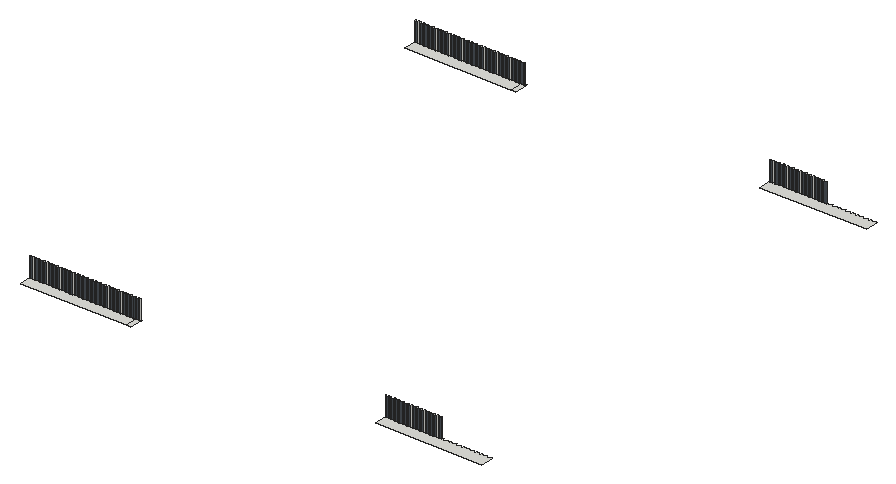
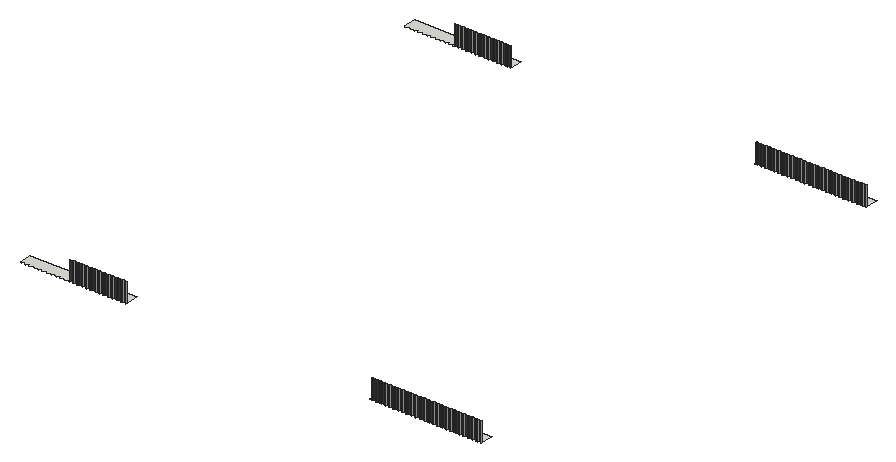
# SketchUp Ruby script. Lengths in inches.
U = 1.inch
M = Sketchup.active_model
def pt(a) = Geom::Point3d.new(a.map { |v| v * U })
def face(e, loops, mat)
  f = e.add_face(loops[0].map { |a| pt(a) })
  loops[1..].each { |l| e.add_face(l.map { |a| pt(a) }).erase! }
  f.material = f.back_material = mat if mat
  f
end
# faces: each face lists its corners as indices into pts; further lists are holes
def faces(e, pts, list, mat = nil) = list.each { |f| face(e, (f[0].is_a?(Array) ? f : [f]).map { |l| l.map { |i| pts[i] } }, mat) }
# xy, xz, yz: faces in a plane at the given z, y or x. An outline is a flat list of corners, or four numbers for a rectangle; further outlines are holes
def ring(l) = l.size == 4 ? [[l[0], l[1]], [l[2], l[1]], [l[2], l[3]], [l[0], l[3]]] : l.each_slice(2).to_a
def flat(e, list, mat, &to3) = list.each { |f| face(e, (f[0].is_a?(Array) ? f : [f]).map { |l| ring(l).map { |u, v| to3.(u, v) } }, mat) }
def xy(e, z, list, mat = nil) = flat(e, list, mat) { |x, y| [x, y, z] }
def xz(e, y, list, mat = nil) = flat(e, list, mat) { |x, z| [x, y, z] }
def yz(e, x, list, mat = nil) = flat(e, list, mat) { |y, z| [x, y, z] }
def lines(e, pts, list) = list.each { |a, b| e.add_line(pt(pts[a]), pt(pts[b])) }
# prism: a flat outline (further loops are holes) pulled along v
def prism(e, loops, v, mat = nil)
  f = face(e, loops, mat); d = Geom::Vector3d.new(v.map { |x| x * U })
  f.pushpull(f.normal.samedirection?(d) ? d.length : -d.length)
end
def box(e, o, s, mat = nil) = prism(e, [[o, [o[0] + s[0], o[1], o[2]], [o[0] + s[0], o[1] + s[1], o[2]], [o[0], o[1] + s[1], o[2]]]], [0, 0, s[2]], mat)
def at(x, y, z, deg = 0) = Geom::Transformation.translation(pt([x, y, z])) * Geom::Transformation.rotation(ORIGIN, Z_AXIS, deg.degrees)
def axes(o, x, y, z) = Geom::Transformation.new([*x, 0, *y, 0, *z, 0, *pt(o).to_a, 1])
def part(name) = M.definitions.add(name)
# library, detail: a bought-in or finely detailed component or shape, given as its bounding box
def library(name, o, s) = part(name).tap { |d| box(d.entities, o, s) }
def detail(e, o, s) = box(e.add_group.entities, o, s)
def put(e, d, t, mat = nil) = e.add_instance(d, t).tap { |i| i.material = mat if mat }
def group(e, t, mat = nil) = e.add_group.tap { |g| g.transformation = t; g.material = mat if mat }.entities
root = M.entities
M.materials.add("[Formica Blue]").color = [73, 80, 86]
xy(root,693.65,[[137.5,412.04,353.97,412.04,353.97,437.1,352.41,437.1,352.41,438.72,349.85,438.72,349.85,437.1,343.52,437.1,343.52,438.72,340.96,438.72,340.96,437.1,334.63,437.1,334.63,438.72,332.07,438.72,332.07,437.1,325.74,437.1,325.74,438.72,323.18,438.72,323.18,437.1,316.85,437.1,316.85,438.72,314.29,438.72,314.29,437.1,307.95,437.1,307.95,438.72,305.4,438.72,305.4,437.1,299.0625,437.1,299.0625,438.72,296.51,438.72,296.51,437.1,290.17,437.1,290.17,438.72,287.61,438.72,287.61,437.1,281.28,437.1,281.28,438.72,278.72,438.72,278.72,437.1,272.39,437.1,272.39,438.72,269.83,438.72,269.83,437.1,263.5,437.1,263.5,438.72,260.94,438.72,260.94,437.1,254.61,437.1,254.61,438.72,252.05,438.72,252.05,437.1,245.72,437.1,245.72,438.72,243.16,438.72,243.16,437.1,236.82,437.1,236.82,438.72,234.27,438.72,234.27,437.1,227.93,437.1,227.93,438.72,225.375,438.72,225.375,437.1,219.04,437.1,219.04,438.72,216.48,438.72,216.48,437.1,210.15,437.1,210.15,438.72,207.59,438.72,207.59,437.1,201.26,437.1,201.26,438.72,198.7,438.72,198.7,437.1,192.37,437.1,192.37,438.72,189.81,438.72,189.81,437.1,183.48,437.1,183.48,438.72,180.92,438.72,180.92,437.1,174.59,437.1,174.59,438.72,172.03,438.72,172.03,437.1,165.69,437.1,165.69,438.72,163.14,438.72,163.14,437.1,156.8,437.1,156.8,438.72,154.24,438.72,154.24,437.1,147.91,437.1,147.91,438.72,143.93,438.72,143.93,437.1,137.6,437.1,137.6,438.72,137.5,438.72],[353.97,412.04,363.73,412.04,363.73,437.1,361.3,437.1,361.3,438.72,358.74,438.72,358.74,437.1,353.97,437.1],[861.9375,412.04,1078.41,412.04,1078.41,437.1,1076.85,437.1,1076.85,438.72,1074.29,438.72,1074.29,437.1,1067.96,437.1,1067.96,438.72,1065.4,438.72,1065.4,437.1,1059.07,437.1,1059.07,438.72,1056.51,438.72,1056.51,437.1,1050.17,437.1,1050.17,438.72,1047.62,438.72,1047.62,437.1,1041.28,437.1,1041.28,438.72,1038.73,438.72,1038.73,437.1,1032.39,437.1,1032.39,438.72,1029.83,438.72,1029.83,437.1,1023.5,437.1,1023.5,438.72,1020.94,438.72,1020.94,437.1,1014.61,437.1,1014.61,438.72,1012.05,438.72,1012.05,437.1,1005.72,437.1,1005.72,438.72,1003.16,438.72,1003.16,437.1,996.83,437.1,996.83,438.72,994.27,438.72,994.27,437.1,987.9375,437.1,987.9375,438.72,985.38,438.72,985.38,437.1,979.04,437.1,979.04,438.72,976.49,438.72,976.49,437.1,970.15,437.1,970.15,438.72,967.6,438.72,967.6,437.1,961.26,437.1,961.26,438.72,958.7,438.72,958.7,437.1,952.37,437.1,952.37,438.72,949.8125,438.72,949.8125,437.1,943.48,437.1,943.48,438.72,940.92,438.72,940.92,437.1,934.59,437.1,934.59,438.72,932.03,438.72,932.03,437.1,925.7,437.1,925.7,438.72,923.14,438.72,923.14,437.1,916.81,437.1,916.81,438.72,914.25,438.72,914.25,437.1,907.91,437.1,907.91,438.72,905.36,438.72,905.36,437.1,899.02,437.1,899.02,438.72,896.47,438.72,896.47,437.1,890.13,437.1,890.13,438.72,887.57,438.72,887.57,437.1,881.24,437.1,881.24,438.72,878.68,438.72,878.68,437.1,872.35,437.1,872.35,438.72,868.37,438.72,868.37,437.1,862.04,437.1,862.04,438.72,861.9375,438.72],[361.3,437.1,363.73,438.72],[137.5,1392.39,353.97,1392.39,353.97,1417.45,352.41,1417.45,352.41,1419.07,349.85,1419.07,349.85,1417.45,343.52,1417.45,343.52,1419.07,340.96,1419.07,340.96,1417.45,334.63,1417.45,334.63,1419.07,332.07,1419.07,332.07,1417.45,325.74,1417.45,325.74,1419.07,323.18,1419.07,323.18,1417.45,316.85,1417.45,316.85,1419.07,314.29,1419.07,314.29,1417.45,307.95,1417.45,307.95,1419.07,305.4,1419.07,305.4,1417.45,299.0625,1417.45,299.0625,1419.07,296.51,1419.07,296.51,1417.45,290.17,1417.45,290.17,1419.07,287.61,1419.07,287.61,1417.45,281.28,1417.45,281.28,1419.07,278.72,1419.07,278.72,1417.45,272.39,1417.45,272.39,1419.07,269.83,1419.07,269.83,1417.45,263.5,1417.45,263.5,1419.07,260.94,1419.07,260.94,1417.45,254.61,1417.45,254.61,1419.07,252.05,1419.07,252.05,1417.45,245.72,1417.45,245.72,1419.07,243.16,1419.07,243.16,1417.45,236.82,1417.45,236.82,1419.07,234.27,1419.07,234.27,1417.45,227.93,1417.45,227.93,1419.07,225.375,1419.07,225.375,1417.45,219.04,1417.45,219.04,1419.07,216.48,1419.07,216.48,1417.45,210.15,1417.45,210.15,1419.07,207.59,1419.07,207.59,1417.45,201.26,1417.45,201.26,1419.07,198.7,1419.07,198.7,1417.45,192.37,1417.45,192.37,1419.07,189.81,1419.07,189.81,1417.45,183.48,1417.45,183.48,1419.07,180.92,1419.07,180.92,1417.45,174.59,1417.45,174.59,1419.07,172.03,1419.07,172.03,1417.45,165.69,1417.45,165.69,1419.07,163.14,1419.07,163.14,1417.45,156.8,1417.45,156.8,1419.07,154.24,1419.07,154.24,1417.45,147.91,1417.45,147.91,1419.07,143.93,1419.07,143.93,1417.45,137.6,1417.45,137.6,1419.07,137.5,1419.07],
  [353.97,1392.39,363.73,1392.39,363.73,1417.45,361.3,1417.45,361.3,1419.07,358.74,1419.07,358.74,1417.45,353.97,1417.45],[861.9375,1392.39,1078.41,1392.39,1078.41,1417.45,1076.85,1417.45,1076.85,1419.07,1074.29,1419.07,1074.29,1417.45,1067.96,1417.45,1067.96,1419.07,1065.4,1419.07,1065.4,1417.45,1059.07,1417.45,1059.07,1419.07,1056.51,1419.07,1056.51,1417.45,1050.17,1417.45,1050.17,1419.07,1047.62,1419.07,1047.62,1417.45,1041.28,1417.45,1041.28,1419.07,1038.73,1419.07,1038.73,1417.45,1032.39,1417.45,1032.39,1419.07,1029.83,1419.07,1029.83,1417.45,1023.5,1417.45,1023.5,1419.07,1020.94,1419.07,1020.94,1417.45,1014.61,1417.45,1014.61,1419.07,1012.05,1419.07,1012.05,1417.45,1005.72,1417.45,1005.72,1419.07,1003.16,1419.07,1003.16,1417.45,996.83,1417.45,996.83,1419.07,994.27,1419.07,994.27,1417.45,987.9375,1417.45,987.9375,1419.07,985.38,1419.07,985.38,1417.45,979.04,1417.45,979.04,1419.07,976.49,1419.07,976.49,1417.45,970.15,1417.45,970.15,1419.07,967.6,1419.07,967.6,1417.45,961.26,1417.45,961.26,1419.07,958.7,1419.07,958.7,1417.45,952.37,1417.45,952.37,1419.07,949.8125,1419.07,949.8125,1417.45,943.48,1417.45,943.48,1419.07,940.92,1419.07,940.92,1417.45,934.59,1417.45,934.59,1419.07,932.03,1419.07,932.03,1417.45,925.7,1417.45,925.7,1419.07,923.14,1419.07,923.14,1417.45,916.81,1417.45,916.81,1419.07,914.25,1419.07,914.25,1417.45,907.91,1417.45,907.91,1419.07,905.36,1419.07,905.36,1417.45,899.02,1417.45,899.02,1419.07,896.47,1419.07,896.47,1417.45,890.13,1417.45,890.13,1419.07,887.57,1419.07,887.57,1417.45,881.24,1417.45,881.24,1419.07,878.68,1419.07,878.68,1417.45,872.35,1417.45,872.35,1419.07,868.37,1419.07,868.37,1417.45,862.04,1417.45,862.04,1419.07,861.9375,1419.07],[361.3,1417.45,363.73,1419.07]])
xz(root,437.1,[[137.6,693.65,143.93,733.125],[147.91,693.65,154.24,733.125],[156.8,693.65,163.14,733.125],[165.69,693.65,172.03,733.125],[174.59,693.65,180.92,733.125],
  [183.48,693.65,189.81,733.125],[192.37,693.65,198.7,733.125],[201.26,693.65,207.59,733.125],[210.15,693.65,216.48,733.125],[219.04,693.65,225.375,733.125],
  [227.93,693.65,234.27,733.125],[236.82,693.65,243.16,733.125],[245.72,693.65,252.05,733.125],[254.61,693.65,260.94,733.125],[263.5,693.65,269.83,733.125],
  [272.39,693.65,278.72,733.125],[281.28,693.65,287.61,733.125],[290.17,693.65,296.51,733.125],[299.0625,693.65,305.4,733.125],[307.95,693.65,314.29,733.125],
  [316.85,693.65,323.18,733.125],[325.74,693.65,332.07,733.125],[334.63,693.65,340.96,733.125],[343.52,693.65,349.85,733.125],[352.41,693.65,358.74,733.125],
  [862.04,693.65,868.37,733.125],[872.35,693.65,878.68,733.125],[881.24,693.65,887.57,733.125],[890.13,693.65,896.47,733.125],[899.02,693.65,905.36,733.125],
  [907.91,693.65,914.25,733.125],[916.81,693.65,923.14,733.125],[925.7,693.65,932.03,733.125],[934.59,693.65,940.92,733.125],[943.48,693.65,949.8125,733.125],
  [952.37,693.65,958.7,733.125],[961.26,693.65,967.6,733.125],[970.15,693.65,976.49,733.125]],"[Formica Blue]")
xz(root,438.72,[[137.5,693.65,137.6,733.125],[861.9375,693.65,862.04,733.125]])
xz(root,438.72,[[143.93,693.65,147.91,733.125],[154.24,693.65,156.8,733.125],[163.14,693.65,165.69,733.125],[172.03,693.65,174.59,733.125],[180.92,693.65,183.48,733.125],
  [189.81,693.65,192.37,733.125],[198.7,693.65,201.26,733.125],[207.59,693.65,210.15,733.125],[216.48,693.65,219.04,733.125],[225.375,693.65,227.93,733.125],
  [234.27,693.65,236.82,733.125],[243.16,693.65,245.72,733.125],[252.05,693.65,254.61,733.125],[260.94,693.65,263.5,733.125],[269.83,693.65,272.39,733.125],
  [278.72,693.65,281.28,733.125],[287.61,693.65,290.17,733.125],[296.51,693.65,299.0625,733.125],[305.4,693.65,307.95,733.125],[314.29,693.65,316.85,733.125],
  [323.18,693.65,325.74,733.125],[332.07,693.65,334.63,733.125],[340.96,693.65,343.52,733.125],[349.85,693.65,352.41,733.125],[358.74,693.65,361.3,733.125],
  [868.37,693.65,872.35,733.125],[878.68,693.65,881.24,733.125],[887.57,693.65,890.13,733.125],[896.47,693.65,899.02,733.125],[905.36,693.65,907.91,733.125],
  [914.25,693.65,916.81,733.125],[923.14,693.65,925.7,733.125],[932.03,693.65,934.59,733.125],[940.92,693.65,943.48,733.125],[949.8125,693.65,952.37,733.125],
  [958.7,693.65,961.26,733.125],[967.6,693.65,970.15,733.125]],"[Formica Blue]")
xz(root,1417.45,[[137.6,693.65,143.93,733.125],[147.91,693.65,154.24,733.125],[156.8,693.65,163.14,733.125],[165.69,693.65,172.03,733.125],[174.59,693.65,180.92,733.125],
  [183.48,693.65,189.81,733.125],[192.37,693.65,198.7,733.125],[201.26,693.65,207.59,733.125],[210.15,693.65,216.48,733.125],[219.04,693.65,225.375,733.125],
  [227.93,693.65,234.27,733.125],[236.82,693.65,243.16,733.125],[245.72,693.65,252.05,733.125],[254.61,693.65,260.94,733.125],[263.5,693.65,269.83,733.125],
  [272.39,693.65,278.72,733.125],[281.28,693.65,287.61,733.125],[290.17,693.65,296.51,733.125],[299.0625,693.65,305.4,733.125],[307.95,693.65,314.29,733.125],
  [316.85,693.65,323.18,733.125],[325.74,693.65,332.07,733.125],[334.63,693.65,340.96,733.125],[343.52,693.65,349.85,733.125],[352.41,693.65,358.74,733.125],
  [862.04,693.65,868.37,733.125],[872.35,693.65,878.68,733.125],[881.24,693.65,887.57,733.125],[890.13,693.65,896.47,733.125],[899.02,693.65,905.36,733.125],
  [907.91,693.65,914.25,733.125],[916.81,693.65,923.14,733.125],[925.7,693.65,932.03,733.125],[934.59,693.65,940.92,733.125],[943.48,693.65,949.8125,733.125],
  [952.37,693.65,958.7,733.125],[961.26,693.65,967.6,733.125],[970.15,693.65,976.49,733.125]],"[Formica Blue]")
xz(root,1419.07,[[137.5,693.65,137.6,733.125],[861.9375,693.65,862.04,733.125]])
xz(root,1419.07,[[143.93,693.65,147.91,733.125],[154.24,693.65,156.8,733.125],[163.14,693.65,165.69,733.125],[172.03,693.65,174.59,733.125],[180.92,693.65,183.48,733.125],
  [189.81,693.65,192.37,733.125],[198.7,693.65,201.26,733.125],[207.59,693.65,210.15,733.125],[216.48,693.65,219.04,733.125],[225.375,693.65,227.93,733.125],
  [234.27,693.65,236.82,733.125],[243.16,693.65,245.72,733.125],[252.05,693.65,254.61,733.125],[260.94,693.65,263.5,733.125],[269.83,693.65,272.39,733.125],
  [278.72,693.65,281.28,733.125],[287.61,693.65,290.17,733.125],[296.51,693.65,299.0625,733.125],[305.4,693.65,307.95,733.125],[314.29,693.65,316.85,733.125],
  [323.18,693.65,325.74,733.125],[332.07,693.65,334.63,733.125],[340.96,693.65,343.52,733.125],[349.85,693.65,352.41,733.125],[358.74,693.65,361.3,733.125],
  [868.37,693.65,872.35,733.125],[878.68,693.65,881.24,733.125],[887.57,693.65,890.13,733.125],[896.47,693.65,899.02,733.125],[905.36,693.65,907.91,733.125],
  [914.25,693.65,916.81,733.125],[923.14,693.65,925.7,733.125],[932.03,693.65,934.59,733.125],[940.92,693.65,943.48,733.125],[949.8125,693.65,952.37,733.125],
  [958.7,693.65,961.26,733.125],[967.6,693.65,970.15,733.125]],"[Formica Blue]")
yz(root,137.6,[[437.1,693.65,438.72,733.125],[1417.45,693.65,1419.07,733.125]])
yz(root,143.93,[[437.1,693.65,438.72,733.125],[1417.45,693.65,1419.07,733.125]])
yz(root,147.91,[[437.1,693.65,438.72,733.125],[1417.45,693.65,1419.07,733.125]])
yz(root,154.24,[[437.1,693.65,438.72,733.125],[1417.45,693.65,1419.07,733.125]])
yz(root,156.8,[[437.1,693.65,438.72,733.125],[1417.45,693.65,1419.07,733.125]])
yz(root,163.14,[[437.1,693.65,438.72,733.125],[1417.45,693.65,1419.07,733.125]])
yz(root,165.69,[[437.1,693.65,438.72,733.125],[1417.45,693.65,1419.07,733.125]])
yz(root,172.03,[[437.1,693.65,438.72,733.125],[1417.45,693.65,1419.07,733.125]])
yz(root,174.59,[[437.1,693.65,438.72,733.125],[1417.45,693.65,1419.07,733.125]])
yz(root,180.92,[[437.1,693.65,438.72,733.125],[1417.45,693.65,1419.07,733.125]])
yz(root,183.48,[[437.1,693.65,438.72,733.125],[1417.45,693.65,1419.07,733.125]])
yz(root,189.81,[[437.1,693.65,438.72,733.125],[1417.45,693.65,1419.07,733.125]])
yz(root,192.37,[[437.1,693.65,438.72,733.125],[1417.45,693.65,1419.07,733.125]])
yz(root,198.7,[[437.1,693.65,438.72,733.125],[1417.45,693.65,1419.07,733.125]])
yz(root,201.26,[[437.1,693.65,438.72,733.125],[1417.45,693.65,1419.07,733.125]])
yz(root,207.59,[[437.1,693.65,438.72,733.125],[1417.45,693.65,1419.07,733.125]])
yz(root,210.15,[[437.1,693.65,438.72,733.125],[1417.45,693.65,1419.07,733.125]])
yz(root,216.48,[[437.1,693.65,438.72,733.125],[1417.45,693.65,1419.07,733.125]])
yz(root,219.04,[[437.1,693.65,438.72,733.125],[1417.45,693.65,1419.07,733.125]])
yz(root,225.375,[[437.1,693.65,438.72,733.125],[1417.45,693.65,1419.07,733.125]])
yz(root,227.93,[[437.1,693.65,438.72,733.125],[1417.45,693.65,1419.07,733.125]])
yz(root,234.27,[[437.1,693.65,438.72,733.125],[1417.45,693.65,1419.07,733.125]])
yz(root,236.82,[[437.1,693.65,438.72,733.125],[1417.45,693.65,1419.07,733.125]])
yz(root,243.16,[[437.1,693.65,438.72,733.125],[1417.45,693.65,1419.07,733.125]])
yz(root,245.72,[[437.1,693.65,438.72,733.125],[1417.45,693.65,1419.07,733.125]])
yz(root,252.05,[[437.1,693.65,438.72,733.125],[1417.45,693.65,1419.07,733.125]])
yz(root,254.61,[[437.1,693.65,438.72,733.125],[1417.45,693.65,1419.07,733.125]])
yz(root,260.94,[[437.1,693.65,438.72,733.125],[1417.45,693.65,1419.07,733.125]])
yz(root,263.5,[[437.1,693.65,438.72,733.125],[1417.45,693.65,1419.07,733.125]])
yz(root,269.83,[[437.1,693.65,438.72,733.125],[1417.45,693.65,1419.07,733.125]])
yz(root,272.39,[[437.1,693.65,438.72,733.125],[1417.45,693.65,1419.07,733.125]])
yz(root,278.72,[[437.1,693.65,438.72,733.125],[1417.45,693.65,1419.07,733.125]])
yz(root,281.28,[[437.1,693.65,438.72,733.125],[1417.45,693.65,1419.07,733.125]])
yz(root,287.61,[[437.1,693.65,438.72,733.125],[1417.45,693.65,1419.07,733.125]])
yz(root,290.17,[[437.1,693.65,438.72,733.125],[1417.45,693.65,1419.07,733.125]])
yz(root,296.51,[[437.1,693.65,438.72,733.125],[1417.45,693.65,1419.07,733.125]])
yz(root,299.0625,[[437.1,693.65,438.72,733.125],[1417.45,693.65,1419.07,733.125]])
yz(root,305.4,[[437.1,693.65,438.72,733.125],[1417.45,693.65,1419.07,733.125]])
yz(root,307.95,[[437.1,693.65,438.72,733.125],[1417.45,693.65,1419.07,733.125]])
yz(root,314.29,[[437.1,693.65,438.72,733.125],[1417.45,693.65,1419.07,733.125]])
yz(root,316.85,[[437.1,693.65,438.72,733.125],[1417.45,693.65,1419.07,733.125]])
yz(root,323.18,[[437.1,693.65,438.72,733.125],[1417.45,693.65,1419.07,733.125]])
yz(root,325.74,[[437.1,693.65,438.72,733.125],[1417.45,693.65,1419.07,733.125]])
yz(root,332.07,[[437.1,693.65,438.72,733.125],[1417.45,693.65,1419.07,733.125]])
yz(root,334.63,[[437.1,693.65,438.72,733.125],[1417.45,693.65,1419.07,733.125]])
yz(root,340.96,[[437.1,693.65,438.72,733.125],[1417.45,693.65,1419.07,733.125]])
yz(root,343.52,[[437.1,693.65,438.72,733.125],[1417.45,693.65,1419.07,733.125]])
yz(root,349.85,[[437.1,693.65,438.72,733.125],[1417.45,693.65,1419.07,733.125]],"[Formica Blue]")
yz(root,352.41,[[437.1,693.65,438.72,733.125],[1417.45,693.65,1419.07,733.125]])
yz(root,358.74,[[437.1,693.65,438.72,733.125],[1417.45,693.65,1419.07,733.125]])
yz(root,361.3,[[437.1,693.65,438.72,733.125],[1417.45,693.65,1419.07,733.125]])
yz(root,862.04,[[437.1,693.65,438.72,733.125],[1417.45,693.65,1419.07,733.125]])
yz(root,868.37,[[437.1,693.65,438.72,733.125],[1417.45,693.65,1419.07,733.125]])
yz(root,872.35,[[437.1,693.65,438.72,733.125],[1417.45,693.65,1419.07,733.125]])
yz(root,878.68,[[437.1,693.65,438.72,733.125],[1417.45,693.65,1419.07,733.125]])
yz(root,881.24,[[437.1,693.65,438.72,733.125],[1417.45,693.65,1419.07,733.125]])
yz(root,887.57,[[437.1,693.65,438.72,733.125],[1417.45,693.65,1419.07,733.125]])
yz(root,890.13,[[437.1,693.65,438.72,733.125],[1417.45,693.65,1419.07,733.125]])
yz(root,896.47,[[437.1,693.65,438.72,733.125],[1417.45,693.65,1419.07,733.125]])
yz(root,899.02,[[437.1,693.65,438.72,733.125],[1417.45,693.65,1419.07,733.125]])
yz(root,905.36,[[437.1,693.65,438.72,733.125],[1417.45,693.65,1419.07,733.125]])
yz(root,907.91,[[437.1,693.65,438.72,733.125],[1417.45,693.65,1419.07,733.125]])
yz(root,914.25,[[437.1,693.65,438.72,733.125],[1417.45,693.65,1419.07,733.125]])
yz(root,916.81,[[437.1,693.65,438.72,733.125],[1417.45,693.65,1419.07,733.125]])
yz(root,923.14,[[437.1,693.65,438.72,733.125],[1417.45,693.65,1419.07,733.125]])
yz(root,925.7,[[437.1,693.65,438.72,733.125],[1417.45,693.65,1419.07,733.125]])
yz(root,932.03,[[437.1,693.65,438.72,733.125],[1417.45,693.65,1419.07,733.125]])
yz(root,934.59,[[437.1,693.65,438.72,733.125],[1417.45,693.65,1419.07,733.125]])
yz(root,940.92,[[437.1,693.65,438.72,733.125],[1417.45,693.65,1419.07,733.125]])
yz(root,943.48,[[437.1,693.65,438.72,733.125],[1417.45,693.65,1419.07,733.125]])
yz(root,949.8125,[[437.1,693.65,438.72,733.125],[1417.45,693.65,1419.07,733.125]])
yz(root,952.37,[[437.1,693.65,438.72,733.125],[1417.45,693.65,1419.07,733.125]])
yz(root,958.7,[[437.1,693.65,438.72,733.125],[1417.45,693.65,1419.07,733.125]])
yz(root,961.26,[[437.1,693.65,438.72,733.125],[1417.45,693.65,1419.07,733.125]])
yz(root,967.6,[[437.1,693.65,438.72,733.125],[1417.45,693.65,1419.07,733.125]])
yz(root,970.15,[[437.1,693.65,438.72,733.125],[1417.45,693.65,1419.07,733.125]])
yz(root,976.49,[[437.1,693.65,438.72,733.125]])
